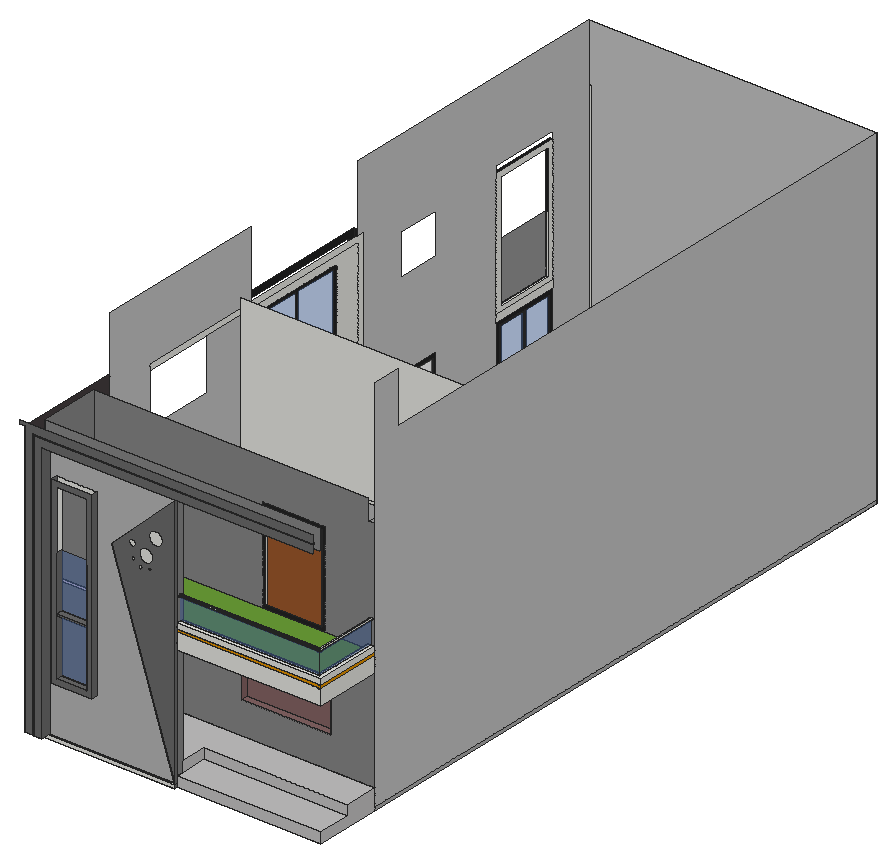
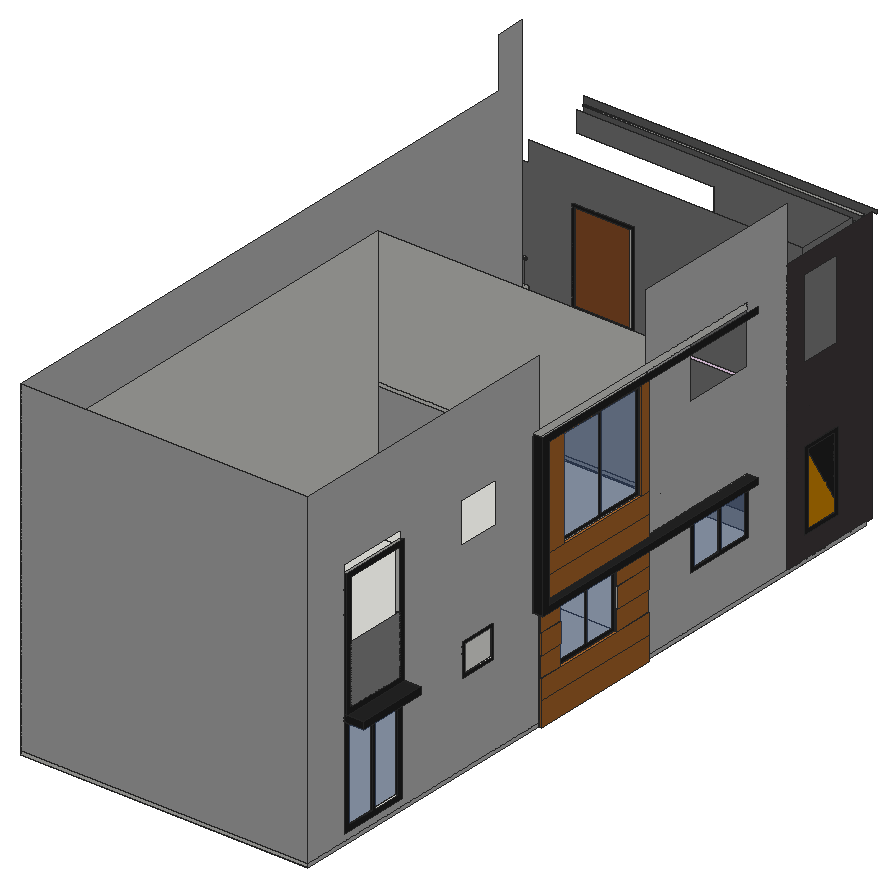
# SketchUp Ruby script. Lengths in inches.
U = 1.inch
M = Sketchup.active_model
def pt(a) = Geom::Point3d.new(a.map { |v| v * U })
def face(e, loops, mat)
  f = e.add_face(loops[0].map { |a| pt(a) })
  loops[1..].each { |l| e.add_face(l.map { |a| pt(a) }).erase! }
  f.material = f.back_material = mat if mat
  f
end
# faces: each face lists its corners as indices into pts; further lists are holes
def faces(e, pts, list, mat = nil) = list.each { |f| face(e, (f[0].is_a?(Array) ? f : [f]).map { |l| l.map { |i| pts[i] } }, mat) }
# xy, xz, yz: faces in a plane at the given z, y or x. An outline is a flat list of corners, or four numbers for a rectangle; further outlines are holes
def ring(l) = l.size == 4 ? [[l[0], l[1]], [l[2], l[1]], [l[2], l[3]], [l[0], l[3]]] : l.each_slice(2).to_a
def flat(e, list, mat, &to3) = list.each { |f| face(e, (f[0].is_a?(Array) ? f : [f]).map { |l| ring(l).map { |u, v| to3.(u, v) } }, mat) }
def xy(e, z, list, mat = nil) = flat(e, list, mat) { |x, y| [x, y, z] }
def xz(e, y, list, mat = nil) = flat(e, list, mat) { |x, z| [x, y, z] }
def yz(e, x, list, mat = nil) = flat(e, list, mat) { |y, z| [x, y, z] }
def lines(e, pts, list) = list.each { |a, b| e.add_line(pt(pts[a]), pt(pts[b])) }
# prism: a flat outline (further loops are holes) pulled along v
def prism(e, loops, v, mat = nil)
  f = face(e, loops, mat); d = Geom::Vector3d.new(v.map { |x| x * U })
  f.pushpull(f.normal.samedirection?(d) ? d.length : -d.length)
end
def box(e, o, s, mat = nil) = prism(e, [[o, [o[0] + s[0], o[1], o[2]], [o[0] + s[0], o[1] + s[1], o[2]], [o[0], o[1] + s[1], o[2]]]], [0, 0, s[2]], mat)
def at(x, y, z, deg = 0) = Geom::Transformation.translation(pt([x, y, z])) * Geom::Transformation.rotation(ORIGIN, Z_AXIS, deg.degrees)
def axes(o, x, y, z) = Geom::Transformation.new([*x, 0, *y, 0, *z, 0, *pt(o).to_a, 1])
def part(name) = M.definitions.add(name)
# library, detail: a bought-in or finely detailed component or shape, given as its bounding box
def library(name, o, s) = part(name).tap { |d| box(d.entities, o, s) }
def detail(e, o, s) = box(e.add_group.entities, o, s)
def put(e, d, t, mat = nil) = e.add_instance(d, t).tap { |i| i.material = mat if mat }
def group(e, t, mat = nil) = e.add_group.tap { |g| g.transformation = t; g.material = mat if mat }.entities
root = M.entities
M.materials.add("[0038_Orange]").color = [221, 143, 0]
M.materials.add("[0117_GhostWhite]").color = [248, 248, 255]
M.materials.add("[0118_Thistle]").color = [216, 191, 216]
M.materials.add("[0119_RosyBrown]").color = [130, 98, 98]
M.materials.add("[0131_Silver]").color = [192, 192, 192]
M.materials.add("[0132_LightGray]").color = [169, 169, 169]
M.materials.add("[0134_DimGray]").color = [105, 105, 105]
M.materials.add("[0135_DarkGray]").color = [35, 35, 35]
M.materials.add("[0136_Charcoal]").color = [35, 35, 35]
M.materials.add("[Asphalt New]").color = [67, 60, 62]
M.materials.add("[Cladding Siding White]").color = [132, 132, 132]
M.materials.add("[Crushed Rock Gravel]").color = [178, 178, 178]
M.materials.add("[Grass Dark Green]").color = [106, 157, 55]
M.materials.add("[Sketchy Scales]").color = [145, 145, 145]
M.materials.add("[Stone Vein Gray]").color = [193, 192, 192]
M.materials.add("[Translucent Glass Blue]").color = [73, 109, 173]
M.materials["[Translucent Glass Blue]"].alpha = 0.5
M.materials.add("[Translucent Glass Gray]").color = [163, 163, 163]
M.materials["[Translucent Glass Gray]"].alpha = 0.5
M.materials.add("[Wood Bamboo]").color = [177, 105, 43]
M.materials.add("[Wood Cherry Original]").color = [152, 86, 42]
xy(root,0,[[72,27,72,936,1092,936,1092,36,582,36,582,27],[72,936,1092,2496],[60,1000.8,72,1476]])
xy(root,12,[[72,0,72,27,132,27,132,0,105,0,105,3,99,3,99,0],[72,27,72,276,96,276,96,60,582,60,582,36,132,36,132,27],[132,27,582,36],[72,276,1092,936],[90,936,1074,2478]])
xy(root,36,[[582,36,1092,156]],"[Stone Vein Gray]")
xy(root,41.4,[[66,2088,72,2340]],"[0135_DarkGray]")
xy(root,59.4,[[66,2106,72,2209],[66,2219,72,2322]])
xy(root,72,[[96,60,582,60,582,156,1092,156,1092,276,96,276]],"[Stone Vein Gray]")
xy(root,92.78,[[69,155.11,72,299.92]],"[0135_DarkGray]")
xy(root,104.78,[[69,167.11,72,287.92]])
xy(root,156.28,[[60,1000.8,63.375,1140],[60,1140,72,1392],[60,1392,63.375,1476]],"[Wood Bamboo]")
xy(root,186.59,[[619.09,276,936.02,300]],"[0119_RosyBrown]")
xy(root,192,[[156,12,300,36]],"[0134_DimGray]")
xy(root,192.28,[[69,552,72,804]],"[0135_DarkGray]")
xy(root,204.28,[[69,564,72,673],[69,683,72,792]],"[0135_DarkGray]")
xy(root,210,[[174,12,282,36]],"[0134_DimGray]")
xy(root,228.28,[[60,1000.8,63.375,1140],[60,1392,63.375,1476]],"[Wood Bamboo]")
xy(root,300.28,[[60,1392,62.5,1476]])
xy(root,300.28,[[60,1000.8,62.5,1140]],"[Wood Bamboo]")
xy(root,310.22,[[72,1684.125,74,1804.125]])
xy(root,360.28,[[69,167.11,72,287.92],[69,564,72,673],[69,683,72,792]],"[0135_DarkGray]")
xy(root,360.28,[[62.5,1140,72,1392]],"[Wood Bamboo]")
xy(root,369.53,[[619.09,276,936.02,300]],"[0119_RosyBrown]")
xy(root,372.28,[[69,552,72,804],[52.84,654.02,51.59,654.13,50.36,654.37,49.16,654.74,48,655.23,46.9,655.84,45.875,656.56,44.93,657.39,44.07,658.31,43.32,659.31,42.67,660.39,42.14,661.53,41.74,662.72,41.46,663.94,41.31,665.19,41.29,666.45,41.4,667.7,41.64,668.93,42.01,670.13,42.5,671.29,43.11,672.38,43.83,673.41,44.66,674.36,45.58,675.21,46.58,675.97,47.66,676.61,48.8,677.14,49.99,677.55,51.21,677.83,52.46,677.98,53.72,678,54.97,677.89,56.2,677.65,57.4,677.28,58.55,676.79,59.65,676.18,60.68,675.45,61.625,674.63,62.48,673.71,63.24,672.7,63.88,671.625,64.41,670.49,64.82,669.3,65.1,668.07,65.25,666.83,65.27,665.57,65.16,664.32,64.92,663.09,64.55,661.89,64.05,660.73,63.44,659.63,62.72,658.61,61.9,657.66,60.98,656.8,59.97,656.05,58.89,655.41,57.76,654.875,56.57,654.47,55.34,654.1875,54.1,654.04],[52.84,870.64,51.59,870.75,50.36,871,49.16,871.36,48,871.86,46.9,872.47,45.875,873.19,44.93,874.02,44.07,874.94,43.32,875.94,42.67,877.02,42.14,878.16,41.74,879.34,41.46,880.57,41.31,881.82,41.29,883.07,41.4,884.32,41.64,885.56,42.01,886.76,42.5,887.91,43.11,889.01,43.83,890.04,44.66,890.98,45.58,891.84,46.58,892.59,47.66,893.24,48.8,893.77,49.99,894.17,51.21,894.46,52.46,894.61,53.72,894.625,54.97,894.51,56.2,894.27,57.4,893.9,58.55,893.41,59.65,892.8,60.68,892.08,61.625,891.25,62.48,890.33,63.24,889.33,63.88,888.25,64.41,887.11,64.82,885.92,65.1,884.7,65.25,883.45,65.27,882.2,65.16,880.95,64.92,879.71,64.55,878.51,64.05,877.36,63.44,876.26,62.72,875.23,61.9,874.28,60.98,873.43,59.97,872.68,58.89,872.03,57.76,871.5,56.57,871.09,55.34,870.8125,54.1,870.66],[62.5,1000.8,72,1476]])
xy(root,372.28,[[69,155.11,72,299.92],[[36,552,36,1500,72,1500,72,1476,62.5,1476,62.5,1000.8,72,1000.8,72,804,69,804,69,552],[52.84,870.64,54.1,870.66,55.34,870.8125,56.57,871.09,57.76,871.5,58.89,872.03,59.97,872.68,60.98,873.43,61.9,874.28,62.72,875.23,63.44,876.26,64.05,877.36,64.55,878.51,64.92,879.71,65.16,880.95,65.27,882.2,65.25,883.45,65.1,884.7,64.82,885.92,64.41,887.11,63.88,888.25,63.24,889.33,62.48,890.33,61.625,891.25,60.68,892.08,59.65,892.8,58.55,893.41,57.4,893.9,56.2,894.27,54.97,894.51,53.72,894.625,52.46,894.61,51.21,894.46,49.99,894.17,48.8,893.77,47.66,893.24,46.58,892.59,45.58,891.84,44.66,890.98,43.83,890.04,43.11,889.01,42.5,887.91,42.01,886.76,41.64,885.56,41.4,884.32,41.29,883.07,41.31,881.82,41.46,880.57,41.74,879.34,42.14,878.16,42.67,877.02,43.32,875.94,44.07,874.94,44.93,874.02,45.875,873.19,46.9,872.47,48,871.86,49.16,871.36,50.36,871,51.59,870.75],[52.84,654.02,54.1,654.04,55.34,654.1875,56.57,654.47,57.76,654.875,58.89,655.41,59.97,656.05,60.98,656.8,61.9,657.66,62.72,658.61,63.44,659.63,64.05,660.73,64.55,661.89,64.92,663.09,65.16,664.32,65.27,665.57,65.25,666.83,65.1,668.07,64.82,669.3,64.41,670.49,63.88,671.625,63.24,672.7,62.48,673.71,61.625,674.63,60.68,675.45,59.65,676.18,58.55,676.79,57.4,677.28,56.2,677.65,54.97,677.89,53.72,678,52.46,677.98,51.21,677.83,49.99,677.55,48.8,677.14,47.66,676.61,46.58,675.97,45.58,675.21,44.66,674.36,43.83,673.41,43.11,672.38,42.5,671.29,42.01,670.13,41.64,668.93,41.4,667.7,41.29,666.45,41.31,665.19,41.46,663.94,41.74,662.72,42.14,661.53,42.67,660.39,43.32,659.31,44.07,658.31,44.93,657.39,45.875,656.56,46.9,655.84,48,655.23,49.16,654.74,50.36,654.37,51.59,654.13]]],"[0135_DarkGray]")
xy(root,376.22,[[66,2106,72,2209],[66,2219,72,2322]],"[0135_DarkGray]")
xy(root,394.22,[[66,2088,72,2340],[30,2202,28.75,2202.07,27.51,2202.26,26.29,2202.59,25.12,2203.04,24,2203.61,22.95,2204.29,21.97,2205.08,21.08,2205.97,20.29,2206.95,19.61,2208,19.04,2209.12,18.59,2210.29,18.26,2211.51,18.07,2212.75,18,2214,18.07,2215.25,18.26,2216.49,18.59,2217.71,19.04,2218.88,19.61,2220,20.29,2221.05,21.08,2222.03,21.97,2222.92,22.95,2223.71,24,2224.39,25.12,2224.96,26.29,2225.41,27.51,2225.74,28.75,2225.93,30,2226,31.25,2225.93,32.49,2225.74,33.71,2225.41,34.88,2224.96,36,2224.39,37.05,2223.71,38.03,2222.92,38.92,2222.03,39.71,2221.05,40.39,2220,40.96,2218.88,41.41,2217.71,41.74,2216.49,41.93,2215.25,42,2214,41.93,2212.75,41.74,2211.51,41.41,2210.29,40.96,2209.12,40.39,2208,39.71,2206.95,38.92,2205.97,38.03,2205.08,37.05,2204.29,36,2203.61,34.88,2203.04,33.71,2202.59,32.49,2202.26,31.25,2202.07]])
xy(root,394.22,[[[0,2088,66,2340],[30,2202,31.25,2202.07,32.49,2202.26,33.71,2202.59,34.88,2203.04,36,2203.61,37.05,2204.29,38.03,2205.08,38.92,2205.97,39.71,2206.95,40.39,2208,40.96,2209.12,41.41,2210.29,41.74,2211.51,41.93,2212.75,42,2214,41.93,2215.25,41.74,2216.49,41.41,2217.71,40.96,2218.88,40.39,2220,39.71,2221.05,38.92,2222.03,38.03,2222.92,37.05,2223.71,36,2224.39,34.88,2224.96,33.71,2225.41,32.49,2225.74,31.25,2225.93,30,2226,28.75,2225.93,27.51,2225.74,26.29,2225.41,25.12,2224.96,24,2224.39,22.95,2223.71,21.97,2222.92,21.08,2222.03,20.29,2221.05,19.61,2220,19.04,2218.88,18.59,2217.71,18.26,2216.49,18.07,2215.25,18,2214,18.07,2212.75,18.26,2211.51,18.59,2210.29,19.04,2209.12,19.61,2208,20.29,2206.95,21.08,2205.97,21.97,2205.08,22.95,2204.29,24,2203.61,25.12,2203.04,26.29,2202.59,27.51,2202.26,28.75,2202.07]]],"[0135_DarkGray]")
xy(root,396.28,[[60,1000.8,72,1476]])
xy(root,396.28,[[36,552,72,552,72,1000.8,60,1000.8,60,1476,36,1476]],"[0135_DarkGray]")
xy(root,406.22,[[72,1684.125,74,1804.125]])
xy(root,410,[[174,12,282,36]],"[0134_DimGray]")
xy(root,418,[[174,12,282,36]],"[0134_DimGray]")
xy(root,418.22,[[60,2088,72,2340]])
xy(root,418.22,[[0,2088,60,2340]],"[0135_DarkGray]")
xy(root,436.22,[[60,2106,72,2322]])
xy(root,436.8,[[582,36,582,60,1068,60,1068,276,1092,276,1092,36]])
xy(root,492,[[582,37,1091,37,1091,276,1068,276,1068,60,582,60]])
xy(root,492,[[582,36,1092,36,1092,276,1091,276,1091,37,582,37]],"[0038_Orange]")
xy(root,492,[[342.64,185.16,339.53,185.55,336.63,186.74,334.14,188.63,332.22,191.1,331,193.99,330.57,197.09,330.96,200.2,332.15,203.1,334.04,205.6,336.51,207.52,339.4,208.74,342.51,209.16,345.61,208.77,348.51,207.59,351.01,205.7,352.93,203.22,354.15,200.33,354.57,197.23,354.18,194.12,353,191.22,351.11,188.73,348.63,186.8,345.74,185.59],[486.64,185.16,483.53,185.55,480.63,186.74,478.14,188.63,476.22,191.1,475,193.99,474.57,197.09,474.96,200.2,476.15,203.1,478.04,205.6,480.51,207.52,483.4,208.74,486.51,209.16,489.61,208.77,492.51,207.59,495.01,205.7,496.93,203.22,498.15,200.33,498.57,197.23,498.18,194.12,497,191.22,495.11,188.73,492.63,186.8,489.74,185.59],[630.64,185.16,627.53,185.55,624.63,186.74,622.14,188.63,620.22,191.1,619,193.99,618.57,197.09,618.96,200.2,620.15,203.1,622.04,205.6,624.51,207.52,627.4,208.74,630.51,209.16,633.61,208.77,636.51,207.59,639.01,205.7,640.93,203.22,642.15,200.33,642.57,197.23,642.18,194.12,641,191.22,639.11,188.73,636.63,186.8,633.74,185.59],[774.64,185.16,771.53,185.55,768.63,186.74,766.14,188.63,764.22,191.1,763,193.99,762.57,197.09,762.96,200.2,764.15,203.1,766.04,205.6,768.51,207.52,771.4,208.74,774.51,209.16,777.61,208.77,780.51,207.59,783.01,205.7,784.93,203.22,786.15,200.33,786.57,197.23,786.18,194.12,785,191.22,783.11,188.73,780.63,186.8,777.74,185.59],[918.64,185.16,915.53,185.55,912.63,186.74,910.14,188.63,908.22,191.1,907,193.99,906.57,197.09,906.96,200.2,908.15,203.1,910.04,205.6,912.51,207.52,915.4,208.74,918.51,209.16,921.61,208.77,924.51,207.59,927.01,205.7,928.93,203.22,930.15,200.33,930.57,197.23,930.18,194.12,929,191.22,927.11,188.73,924.63,186.8,921.74,185.59]],"[0117_GhostWhite]")
xy(root,492,[[[96,60,1068,276],[918.64,185.16,921.74,185.59,924.63,186.8,927.11,188.73,929,191.22,930.18,194.12,930.57,197.23,930.15,200.33,928.93,203.22,927.01,205.7,924.51,207.59,921.61,208.77,918.51,209.16,915.4,208.74,912.51,207.52,910.04,205.6,908.15,203.1,906.96,200.2,906.57,197.09,907,193.99,908.22,191.1,910.14,188.63,912.63,186.74,915.53,185.55],[774.64,185.16,777.74,185.59,780.63,186.8,783.11,188.73,785,191.22,786.18,194.12,786.57,197.23,786.15,200.33,784.93,203.22,783.01,205.7,780.51,207.59,777.61,208.77,774.51,209.16,771.4,208.74,768.51,207.52,766.04,205.6,764.15,203.1,762.96,200.2,762.57,197.09,763,193.99,764.22,191.1,766.14,188.63,768.63,186.74,771.53,185.55],[630.64,185.16,633.74,185.59,636.63,186.8,639.11,188.73,641,191.22,642.18,194.12,642.57,197.23,642.15,200.33,640.93,203.22,639.01,205.7,636.51,207.59,633.61,208.77,630.51,209.16,627.4,208.74,624.51,207.52,622.04,205.6,620.15,203.1,618.96,200.2,618.57,197.09,619,193.99,620.22,191.1,622.14,188.63,624.63,186.74,627.53,185.55],[486.64,185.16,489.74,185.59,492.63,186.8,495.11,188.73,497,191.22,498.18,194.12,498.57,197.23,498.15,200.33,496.93,203.22,495.01,205.7,492.51,207.59,489.61,208.77,486.51,209.16,483.4,208.74,480.51,207.52,478.04,205.6,476.15,203.1,474.96,200.2,474.57,197.09,475,193.99,476.22,191.1,478.14,188.63,480.63,186.74,483.53,185.55],[342.64,185.16,345.74,185.59,348.63,186.8,351.11,188.73,353,191.22,354.18,194.12,354.57,197.23,354.15,200.33,352.93,203.22,351.01,205.7,348.51,207.59,345.61,208.77,342.51,209.16,339.4,208.74,336.51,207.52,334.04,205.6,332.15,203.1,330.96,200.2,330.57,197.09,331,193.99,332.22,191.1,334.14,188.63,336.63,186.74,339.53,185.55]]],"[0118_Thistle]")
xy(root,504,[[582,37,582,60,1068,60,1068,276,1091,276,1091,37]])
xy(root,504,[[582,36,582,37,1091,37,1091,276,1092,276,1092,36]],"[0038_Orange]")
xy(root,504,[[96,60,1068,276]],"[Grass Dark Green]")
xy(root,516,[[705.53,276,902.41,278]])
xy(root,522,[[582,36,1092,36,1092,276,1080,276,1080,48,582,48],[582,48,1080,48,1080,276,1068,276,1068,60,582,60]])
xy(root,540.28,[[60,1032,72,1380]],"[Wood Bamboo]")
xz(root,0,[[72,12,99,12,99,969,1092,969,1092,996,56,996,56,984,72,984],[105,12,132,12,132,936,1092,936,1092,963,105,963]],"[0134_DimGray]")
xz(root,3,[[99,12,105,12,105,963,1092,963,1092,969,99,969]])
xz(root,12,[[[156,192,300,840],[174,210,282,822]],[174,410,282,418]],"[0134_DimGray]")
xz(root,27,[[72,0,582,12]])
xz(root,27,[[[582,12,582,912,357.71,698.8],[513.45,744.7,510.95,744.97,508.5,745.49,506.11,746.27,503.8125,747.29,501.64,748.55,499.61,750.03,497.74,751.71,496.0625,753.58,494.59,755.61,493.33,757.79,492.3125,760.09,491.54,762.48,491.02,764.93,490.76,767.43,490.76,769.94,491.02,772.44,491.55,774.9,492.33,777.29,493.35,779.58,494.61,781.76,496.09,783.79,497.77,785.65,499.64,787.33,501.67,788.81,503.85,790.0625,506.14,791.08,508.53,791.86,510.99,792.375,513.49,792.64,516,792.63,518.5,792.37,520.96,791.85,523.35,791.07,525.64,790.04,527.8125,788.79,529.85,787.31,531.71,785.625,533.39,783.76,534.86,781.72,536.12,779.55,537.14,777.25,537.91,774.86,538.43,772.4,538.69,769.91,538.69,767.39,538.43,764.9,537.9,762.4375,537.125,760.05,536.1,757.76,534.84,755.58,533.37,753.55,531.68,751.68,529.82,750.01,527.78,748.53,525.6,747.28,523.31,746.26,520.92,745.48,518.46,744.96,515.96,744.7],[480.75,679.13,478.24,679.23,475.76,679.59,473.32,680.2,470.96,681.07,468.71,682.18,466.58,683.51,464.61,685.07,462.8,686.82,461.2,688.75,459.8,690.83,458.625,693.05,457.69,695.39,457.01,697.8,456.58,700.28,456.41,702.78,456.5,705.29,456.86,707.78,457.48,710.22,458.34,712.57,459.45,714.83,460.79,716.96,462.34,718.93,464.09,720.73,466.02,722.34,468.11,723.74,470.33,724.91,472.66,725.85,475.08,726.53,477.55,726.96,480.06,727.13,482.57,727.03,485.06,726.68,487.49,726.0625,489.85,725.19,492.11,724.09,494.23,722.75,496.21,721.2,498.01,719.45,499.62,717.52,501.02,715.43,502.1875,713.21,503.12,710.875,503.81,708.46,504.24,705.98,504.4,703.48,504.31,700.97,503.95,698.48,503.34,696.04,502.47,693.6875,501.36,691.43,500.02,689.31,498.47,687.33,496.72,685.53,494.79,683.92,492.71,682.52,490.48,681.35,488.15,680.41,485.73,679.73,483.26,679.3],[432.01,715.13,430.75,715.14,429.51,715.28,428.28,715.55,427.09,715.94,425.94,716.46,424.86,717.09,423.85,717.84,422.92,718.68,422.08,719.62,421.35,720.64,420.73,721.73,420.22,722.88,419.84,724.08,419.59,725.31,419.46,726.56,419.47,727.82,419.61,729.06,419.875,730.29,420.27,731.48,420.79,732.63,421.42,733.71,422.17,734.72,423.01,735.65,423.95,736.49,424.97,737.22,426.0625,737.84,427.21,738.35,428.41,738.73,429.64,738.98,430.89,739.11,432.15,739.1,433.39,738.96,434.62,738.69,435.8125,738.3,436.96,737.78,438.04,737.15,439.05,736.4,439.98,735.56,440.82,734.62,441.55,733.6,442.17,732.51,442.68,731.36,443.06,730.16,443.3125,728.93,443.4375,727.68,443.43,726.42,443.29,725.18,443.02,723.95,442.63,722.76,442.11,721.61,441.48,720.53,440.73,719.52,439.89,718.59,438.95,717.75,437.93,717.02,436.84,716.4,435.6875,715.89,434.49,715.51,433.26,715.26],[434.44,671.83,433.57,671.94,432.72,672.16,431.9,672.49,431.13,672.91,430.42,673.43,429.78,674.03,429.22,674.7,428.75,675.45,428.375,676.24,428.1,677.08,427.9375,677.94,427.88,678.82,427.9375,679.7,428.1,680.56,428.375,681.4,428.75,682.19,429.22,682.93,429.78,683.61,430.42,684.21,431.13,684.73,431.9,685.15,432.72,685.48,433.57,685.7,434.44,685.81,435.32,685.81,436.19,685.7,437.05,685.48,437.86,685.15,438.63,684.73,439.35,684.21,439.99,683.61,440.55,682.93,441.02,682.19,441.39,681.4,441.66,680.56,441.83,679.7,441.88,678.82,441.83,677.94,441.66,677.08,441.39,676.24,441.02,675.45,440.55,674.7,439.99,674.03,439.35,673.43,438.63,672.91,437.86,672.49,437.05,672.16,436.19,671.94,435.32,671.83],[460.54,652.35,459.66,652.46,458.8125,652.68,458,653,457.22,653.43,456.51,653.95,455.875,654.55,455.3125,655.22,454.84,655.97,454.47,656.76,454.2,657.6,454.03,658.46,453.98,659.34,454.03,660.22,454.2,661.08,454.47,661.92,454.84,662.71,455.3125,663.45,455.875,664.13,456.51,664.73,457.22,665.25,458,665.67,458.8125,666,459.66,666.21,460.54,666.32,461.42,666.32,462.29,666.21,463.14,666,463.96,665.67,464.73,665.25,465.4375,664.73,466.08,664.13,466.64,663.45,467.11,662.71,467.48,661.92,467.76,661.08,467.92,660.22,467.98,659.34,467.92,658.46,467.76,657.6,467.48,656.76,467.11,655.97,466.64,655.22,466.08,654.55,465.4375,653.95,464.73,653.43,463.96,653,463.14,652.68,462.29,652.46,461.42,652.35],[492.87,657.98,492.24,658.01,491.62,658.11,491.01,658.28,490.43,658.5,489.87,658.79,489.34,659.13,488.85,659.53,488.41,659.97,488.01,660.46,487.67,660.99,487.39,661.55,487.16,662.13,487,662.74,486.9,663.36,486.87,663.99,486.91,664.61,487.01,665.24,487.17,665.84,487.39,666.43,487.68,666.99,488.02,667.51,488.42,668,488.86,668.44,489.35,668.84,489.88,669.18,490.44,669.46,491.03,669.6875,491.63,669.85,492.25,669.95,492.88,669.98,493.51,669.95,494.13,669.85,494.73,669.68,495.32,669.46,495.88,669.17,496.41,668.83,496.89,668.43,497.34,667.99,497.73,667.5,498.07,666.97,498.36,666.41,498.58,665.83,498.74,665.22,498.84,664.6,498.87,663.97,498.84,663.35,498.74,662.72,498.58,662.12,498.35,661.53,498.07,660.97,497.72,660.45,497.33,659.96,496.88,659.52,496.39,659.12,495.87,658.78,495.31,658.5,494.72,658.27,494.11,658.11,493.49,658.01]]],"[0134_DimGray]")
xz(root,36,[[582,12,357.71,698.8,582,912],[[156,192,300,840],[174,210,282,822]],[174,410,282,418],[582,436.8,1092,492],[582,504,1092,522]])
xz(root,36,[[[132,12,582,12,357.71,698.8,582,912,582,936,132,936],[156,192,300,840]]],"[Crushed Rock Gravel]")
xz(root,36,[[582,0,1092,36]],"[Stone Vein Gray]")
xz(root,36,[[174,210,282,410],[174,418,282,610]],"[Translucent Glass Blue]")
xz(root,37,[[582,492,1091,504]],"[0038_Orange]")
xz(root,48,[[582,600,1080,606]])
xz(root,48,[[582,522,1080,600]],"[Translucent Glass Blue]")
xz(root,60,[[96,12,582,72],[582,436.8,1068,492],[582,504,1068,522]])
xz(root,60,[[96,72,582,492],[96,504,96,984,1068,984,1068,912,582,912,582,504]],"[Cladding Siding White]")
xz(root,155.11,[[69,92.78,72,372.28]],"[0135_DarkGray]")
xz(root,156,[[582,36,1092,72]],"[Stone Vein Gray]")
xz(root,167.11,[[69,104.78,72,360.28]],"[0135_DarkGray]")
xz(root,276,[[96,12,1092,72],[1068,436.8,1092,492],[1091,492,1092,504],[1068,504,1092,522],[1080,600,1078.45,600.2,1077,600.8,1075.76,601.76,1074.8,603,1074.2,604.45,1074,606,1074.2,607.55,1074.8,609,1075.76,610.24,1077,611.2,1078.45,611.8,1080,612,1081.55,611.8,1083,611.2,1084.24,610.24,1085.2,609,1085.8,607.55,1086,606,1085.8,604.45,1085.2,603,1084.24,601.76,1083,600.8,1081.55,600.2]])
xz(root,276,[[[693.53,504,914.41,839.4375],[705.53,516,902.41,827.4375]]],"[0136_Charcoal]")
xz(root,276,[[[96,72,1092,72,1092,436.8,1068,436.8,1068,492,96,492],[619.09,186.59,936.02,369.53]],[[96,504,693.53,504,693.53,839.4375,914.41,839.4375,914.41,504,1068,504,1068,522,1092,522,1092,912,1068,912,1068,984,96,984],[1080,600,1078.45,600.2,1077,600.8,1075.76,601.76,1074.8,603,1074.2,604.45,1074,606,1074.2,607.55,1074.8,609,1075.76,610.24,1077,611.2,1078.45,611.8,1080,612,1081.55,611.8,1083,611.2,1084.24,610.24,1085.2,609,1085.8,607.55,1086,606,1085.8,604.45,1085.2,603,1084.24,601.76,1083,600.8,1081.55,600.2]]],"[Cladding Siding White]")
xz(root,278,[[705.53,516,902.41,827.4375]],"[Wood Cherry Original]")
xz(root,287.92,[[69,104.78,72,360.28]],"[0135_DarkGray]")
xz(root,299.92,[[69,92.78,72,372.28]],"[0135_DarkGray]")
xz(root,300,[[619.09,186.59,936.02,369.53]],"[0119_RosyBrown]")
xz(root,552,[[69,192.28,72,372.28],[36,372.28,72,396.28]],"[0135_DarkGray]")
xz(root,564,[[69,204.28,72,360.28]],"[0135_DarkGray]")
xz(root,673,[[69,204.28,72,360.28]],"[0135_DarkGray]")
xz(root,683,[[69,204.28,72,360.28]],"[0135_DarkGray]")
xz(root,792,[[69,204.28,72,360.28]],"[0135_DarkGray]")
xz(root,804,[[69,192.28,72,372.28]],"[0135_DarkGray]")
xz(root,936,[[90,492,1074,504],[90,504,1074,984]])
xz(root,1000.8,[[60,0,72,0,72,372.28,62.5,372.28,62.5,300.28,60,300.28,60,228.28,63.375,228.28,63.375,156.28,60,156.28],[60,396.28,72,915.4]],"[Wood Bamboo]")
xz(root,1032,[[60,540.28,72,891.4]],"[Wood Bamboo]")
xz(root,1140,[[63.375,156.28,63.375,228.28,60,228.28,60,300.28,62.5,300.28,62.5,360.28,72,360.28,72,156.28]])
xz(root,1380,[[60,540.28,72,891.4]],"[Wood Bamboo]")
xz(root,1392,[[63.375,156.28,72,156.28,72,360.28,62.5,360.28,62.5,300.28,60,300.28,60,228.28,63.375,228.28]],"[Wood Bamboo]")
xz(root,1476,[[60,396.28,72,915.4]])
xz(root,1476,[[36,396.28,60,915.4]],"[0135_DarkGray]")
xz(root,1476,[[60,0,60,156.28,63.375,156.28,63.375,228.28,60,228.28,60,300.28,62.5,300.28,62.5,372.28,72,372.28,72,0]],"[Wood Bamboo]")
xz(root,1500,[[36,372.28,72,939.4]],"[0135_DarkGray]")
xz(root,1684.125,[[72,310.22,74,406.22]])
xz(root,1804.125,[[72,310.22,74,406.22]])
xz(root,2088,[[66,41.4,72,394.22],[0,394.22,72,418.22],[60,418.22,72,867.4]],"[0135_DarkGray]")
xz(root,2106,[[60,436.22,72,642.81]])
xz(root,2106,[[66,59.4,72,376.22]],"[0135_DarkGray]")
xz(root,2209,[[66,59.4,72,376.22]],"[0135_DarkGray]")
xz(root,2219,[[66,59.4,72,376.22]],"[0135_DarkGray]")
xz(root,2322,[[60,436.22,72,642.81]])
xz(root,2322,[[66,59.4,72,376.22]],"[0135_DarkGray]")
xz(root,2340,[[66,41.4,72,394.22],[0,394.22,72,418.22],[60,418.22,72,867.4]],"[0135_DarkGray]")
xz(root,2478,[[90,12,96.25,984]])
xz(root,2496,[[72,0,1092,12]])
xz(root,2496,[[72,12,1092,1176]],"[0131_Silver]")
yz(root,0,[[2088,394.22,2340,418.22]],"[0135_DarkGray]")
yz(root,36,[[552,372.28,552,396.28,1476,396.28,1476,915.4,552,915.4,552,939.4,1500,939.4,1500,372.28]],"[0135_DarkGray]")
yz(root,60,[[[2088,418.22,2340,867.4],[2106,436.22,2322,849.4]]],"[0135_DarkGray]")
yz(root,60,[[2106,436.22,2322,642.81]],"[Sketchy Scales]")
yz(root,60,[[1000.8,0,1476,84.28],[1000.8,84.28,1476,156.28],[1000.8,228.28,1140,300.28],[1392,228.28,1476,300.28],[1000.8,396.28,1476,468.28],
  [1000.8,468.28,1476,540.28],[1000.8,540.28,1000.8,915.4,1476,915.4,1476,540.28,1380,540.28,1380,891.4,1032,891.4,1032,540.28]],"[Wood Bamboo]")
yz(root,62.5,[[1000.8,300.28,1000.8,372.28,1476,372.28,1476,300.28,1392,300.28,1392,360.28,1140,360.28,1140,300.28]],"[Wood Bamboo]")
yz(root,63.375,[[1000.8,156.28,1140,228.28],[1392,156.28,1476,228.28]],"[Wood Bamboo]")
yz(root,66,[[[2088,41.4,2340,394.22],[2219,59.4,2322,376.22],[2106,59.4,2209,376.22]]],"[0135_DarkGray]")
yz(root,69,[[[155.11,92.78,299.92,372.28],[167.11,104.78,287.92,360.28]],[[552,192.28,804,372.28],[683,204.28,792,360.28],[564,204.28,673,360.28]]],"[0135_DarkGray]")
yz(root,72,[[[1000.8,0,1476,372.28],[1140,156.28,1392,360.28]],[[155.11,92.78,299.92,372.28],[167.11,104.78,287.92,360.28]],[552,372.28,1500,372.28,1500,939.4,552,939.4,552,915.4,1476,915.4,1476,396.28,552,396.28],[2088,394.22,2340,418.22],[[1000.8,396.28,1476,915.4],[1032,540.28,1380,891.4]],
  [[2088,418.22,2340,867.4],[2106,436.22,2322,849.4]]])
yz(root,72,[[167.11,104.78,167.11,153.72,287.92,360.28,287.92,104.78]],"[0038_Orange]")
yz(root,72,[[27,0,1000.8,12],[1476,0,2496,12],[378,12,378,1176,1000.8,1176,1000.8,939.4,552,939.4,552,735.4,804,735.4,804,915.4,1000.8,915.4,1000.8,396.28,552,396.28,552,192.28,804,192.28,804,372.28,1000.8,372.28,1000.8,12],[[1476,12,1476,372.28,1500,372.28,1500,939.4,1476,939.4,1476,1176,2496,1176,2496,12],[2088,41.4,2340,891.4],[1666.125,723.4,1822.125,867.4],[1672.125,298.22,1816.125,418.22]]],"[0131_Silver]")
yz(root,72,[[167.11,153.72,167.11,360.28,287.92,360.28],[[1140,156.28,1392,360.28],[1271,168.28,1380,348.28],[1152,168.28,1261,348.28]],[[1672.125,298.22,1816.125,418.22],[1684.125,310.22,1804.125,406.22]],[[1032,540.28,1380,891.4],[1044,552.28,1201,879.4],[1211,552.28,1368,879.4]]],"[0135_DarkGray]")
yz(root,72,[[[0,12,378,984],[155.11,92.78,299.92,372.28],[155.11,635.9,299.92,915.4]]],"[Asphalt New]")
yz(root,72,[[2106,59.4,2209,376.22],[2219,59.4,2322,376.22],[1152,168.28,1261,348.28],[1271,168.28,1380,348.28],[564,204.28,673,360.28],
  [683,204.28,792,360.28],[1044,552.28,1201,879.4],[1211,552.28,1368,879.4]],"[Translucent Glass Blue]")
yz(root,74,[[1684.125,310.22,1804.125,406.22]],"[Translucent Glass Gray]")
yz(root,96,[[60,12,276,72]])
yz(root,96,[[60,72,276,492],[60,504,276,984]],"[Cladding Siding White]")
yz(root,99,[[0,12,3,969]])
yz(root,105,[[0,12,3,963]])
yz(root,132,[[0,12,36,936]],"[0134_DimGray]")
yz(root,156,[[12,192,36,840]],"[0134_DimGray]")
yz(root,174,[[12,410,36,418]])
yz(root,174,[[12,210,36,410],[12,418,36,610]],"[0134_DimGray]")
yz(root,282,[[12,410,36,418]])
yz(root,282,[[12,210,36,410],[12,418,36,610]],"[0134_DimGray]")
yz(root,300,[[12,192,36,840]],"[0134_DimGray]")
yz(root,582,[[36,12,60,36],[36,436.8,60,492],[36,492,37,504],[36,504,60,522]])
yz(root,582,[[27,0,36,12],[27,12,36,912]],"[0134_DimGray]")
yz(root,582,[[36,36,60,436.8],[[36,522,60,912],[48,600,46.45,600.2,45,600.8,43.76,601.76,42.8,603,42.2,604.45,42,606,42.2,607.55,42.8,609,43.76,610.24,45,611.2,46.45,611.8,48,612,49.55,611.8,51,611.2,52.24,610.24,53.2,609,53.8,607.55,54,606,53.8,604.45,53.2,603,52.24,601.76,51,600.8,49.55,600.2]]],"[Cladding Siding White]")
yz(root,582,[[60,36,156,72]],"[Stone Vein Gray]")
yz(root,619.09,[[276,186.59,300,369.53]],"[0119_RosyBrown]")
yz(root,705.53,[[276,516,278,827.4375]])
yz(root,902.41,[[276,516,278,827.4375]])
yz(root,936.02,[[276,186.59,300,369.53]],"[0119_RosyBrown]")
yz(root,1068,[[60,436.8,276,492],[60,504,276,522]])
yz(root,1074,[[936,12,2478,984]])
yz(root,1080,[[48,600,276,606]])
yz(root,1080,[[48,522,276,600]],"[Translucent Glass Blue]")
yz(root,1091,[[37,492,276,504]],"[0038_Orange]")
yz(root,1092,[[36,436.8,276,492],[36,504,276,522]])
yz(root,1092,[[276,12,2496,12,2496,1176,378,1176,378,1356,276,1356]],"[0131_Silver]")
yz(root,1092,[[276,0,2496,12]],"[0132_LightGray]")
yz(root,1092,[[36,0,276,0,276,72,156,72,156,36,36,36]],"[Stone Vein Gray]")
p = [[357.71,36,698.8],[582,36,12],[582,27,12],[357.71,27,698.8],[1080,48,600],[1081.55,46.45,600.2],
  [582,46.45,600.2],[582,48,600],[1080,276,600],[1081.55,276,600.2],[1078.45,49.55,600.2],[582,49.55,600.2],
  [1078.45,276,600.2],[1083,45,600.8],[582,45,600.8],[1083,276,600.8],[1077,51,600.8],[582,51,600.8],
  [1077,276,600.8],[1084.24,43.76,601.76],[582,43.76,601.76],[1084.24,276,601.76],[1075.76,52.24,601.76],[582,52.24,601.76],
  [1075.76,276,601.76],[1085.2,42.8,603],[582,42.8,603],[1085.2,276,603],[1074.8,53.2,603],[582,53.2,603],
  [1074.8,276,603],[1085.8,42.2,604.45],[582,42.2,604.45],[1085.8,276,604.45],[1074.2,53.8,604.45],[582,53.8,604.45],
  [1074.2,276,604.45],[1086,42,606],[582,42,606],[1086,276,606],[1074,54,606],[582,54,606],
  [1074,276,606],[72,276,492],[96,276,492],[90,936,504],[72,936,504]]
faces(root,p,[[0,1,2,3]],"[0134_DimGray]")
faces(root,p,[[4,5,6,7],[8,9,5,4],[10,4,7,11],[12,8,4,10],[5,13,14,6],[9,15,13,5],[16,10,11,17],[18,12,10,16],
  [13,19,20,14],[15,21,19,13],[22,16,17,23],[24,18,16,22],[19,25,26,20],[21,27,25,19],[28,22,23,29],[30,24,22,28],
  [25,31,32,26],[27,33,31,25],[34,28,29,35],[36,30,28,34],[31,37,38,32],[33,39,37,31],[40,34,35,41],[42,36,34,40]])
lines(root,p,[[43,44],[45,46]])
